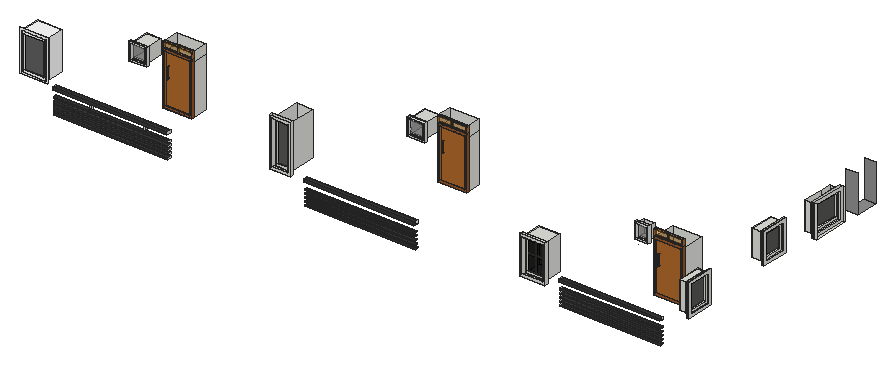
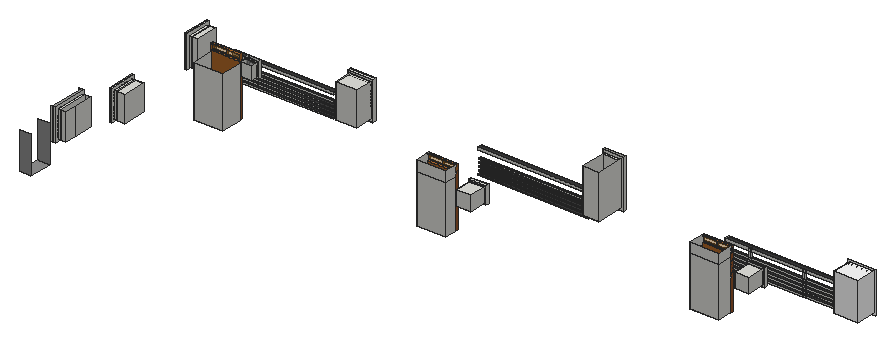
# SketchUp Ruby script. Lengths in inches.
U = 1.inch
M = Sketchup.active_model
def pt(a) = Geom::Point3d.new(a.map { |v| v * U })
def face(e, loops, mat)
  f = e.add_face(loops[0].map { |a| pt(a) })
  loops[1..].each { |l| e.add_face(l.map { |a| pt(a) }).erase! }
  f.material = f.back_material = mat if mat
  f
end
# faces: each face lists its corners as indices into pts; further lists are holes
def faces(e, pts, list, mat = nil) = list.each { |f| face(e, (f[0].is_a?(Array) ? f : [f]).map { |l| l.map { |i| pts[i] } }, mat) }
# xy, xz, yz: faces in a plane at the given z, y or x. An outline is a flat list of corners, or four numbers for a rectangle; further outlines are holes
def ring(l) = l.size == 4 ? [[l[0], l[1]], [l[2], l[1]], [l[2], l[3]], [l[0], l[3]]] : l.each_slice(2).to_a
def flat(e, list, mat, &to3) = list.each { |f| face(e, (f[0].is_a?(Array) ? f : [f]).map { |l| ring(l).map { |u, v| to3.(u, v) } }, mat) }
def xy(e, z, list, mat = nil) = flat(e, list, mat) { |x, y| [x, y, z] }
def xz(e, y, list, mat = nil) = flat(e, list, mat) { |x, z| [x, y, z] }
def yz(e, x, list, mat = nil) = flat(e, list, mat) { |y, z| [x, y, z] }
def lines(e, pts, list) = list.each { |a, b| e.add_line(pt(pts[a]), pt(pts[b])) }
# prism: a flat outline (further loops are holes) pulled along v
def prism(e, loops, v, mat = nil)
  f = face(e, loops, mat); d = Geom::Vector3d.new(v.map { |x| x * U })
  f.pushpull(f.normal.samedirection?(d) ? d.length : -d.length)
end
def box(e, o, s, mat = nil) = prism(e, [[o, [o[0] + s[0], o[1], o[2]], [o[0] + s[0], o[1] + s[1], o[2]], [o[0], o[1] + s[1], o[2]]]], [0, 0, s[2]], mat)
def at(x, y, z, deg = 0) = Geom::Transformation.translation(pt([x, y, z])) * Geom::Transformation.rotation(ORIGIN, Z_AXIS, deg.degrees)
def axes(o, x, y, z) = Geom::Transformation.new([*x, 0, *y, 0, *z, 0, *pt(o).to_a, 1])
def part(name) = M.definitions.add(name)
# library, detail: a bought-in or finely detailed component or shape, given as its bounding box
def library(name, o, s) = part(name).tap { |d| box(d.entities, o, s) }
def detail(e, o, s) = box(e.add_group.entities, o, s)
def put(e, d, t, mat = nil) = e.add_instance(d, t).tap { |i| i.material = mat if mat }
def group(e, t, mat = nil) = e.add_group.tap { |g| g.transformation = t; g.material = mat if mat }.entities
root = M.entities
M.materials.add("Generic").color = [145, 145, 145]
M.materials.add("[Color M00]").color = [255, 255, 255]
M.materials.add("[Color M07]").color = [58, 58, 58]
M.materials.add("[Color M08]").color = [45, 45, 45]
M.materials.add("[Translucent Glass Dark Green]").color = [168, 100, 12]
M.materials["[Translucent Glass Dark Green]"].alpha = 0.5
M.materials.add("[Translucent Glass Gray]").color = [0, 0, 0]
M.materials["[Translucent Glass Gray]"].alpha = 0.62
M.materials.add("[Translucent Glass Gray]1").color = [128, 128, 128]
M.materials["[Translucent Glass Gray]1"].alpha = 0.5
M.materials.add("[Wood Bamboo]").color = [177, 105, 43]
M.materials.add("[Wood Cherry Original]").color = [152, 86, 42]
c1 = part("Group\#10")
xy(c1.entities,0,[[0,1.08,55.8125,6.01]],"[Wood Cherry Original]")
xy(c1.entities,3.96,[[3.96,1.08,51.86,3.01]],"[Wood Bamboo]")
xy(c1.entities,51.66,[[8.63,0,9.88,3.01]],"[Color M08]")
xy(c1.entities,52.54,[[8.63,0.6875,9.88,3.01]],"[Color M08]")
xy(c1.entities,71.82,[[8.63,0.6875,9.88,3.01]],"[Color M08]")
xy(c1.entities,72.69,[[8.63,0,9.88,3.01]],"[Color M08]")
xy(c1.entities,97.36,[[3.96,1.08,51.86,3.01]],"[Wood Bamboo]")
xy(c1.entities,101.3125,[[0,1.08,55.8125,6.01]],"[Wood Bamboo]")
xy(c1.entities,102.55,[[1.23,1.08,27.29,3.01],[27.29,1.08,28.52,1.95],[28.52,1.08,54.58,3.01]],"[Wood Bamboo]")
xy(c1.entities,112.31,[[1.23,1.08,1.23,3.01,27.29,3.01,27.29,1.95,28.52,1.95,28.52,3.01,54.58,3.01,54.58,1.08]],"[Wood Bamboo]")
xy(c1.entities,113.54,[[0,1.08,55.8125,6.01]],"[Wood Bamboo]")
xz(c1.entities,0,[[8.63,51.66,9.88,72.69]],"[Color M08]")
xz(c1.entities,0.6875,[[8.63,52.54,9.88,71.82]])
xz(c1.entities,1.08,[[0,101.3125,55.8125,102.55],[0,102.55,1.23,102.55,1.23,112.31,54.58,112.31,54.58,102.55,55.8125,102.55,55.8125,113.54,0,113.54]],"[Wood Bamboo]")
xz(c1.entities,1.08,[[[0,0,55.8125,101.3125],[3.96,3.96,51.86,97.36]]],"[Wood Cherry Original]")
xz(c1.entities,1.95,[[27.29,102.55,28.52,112.31]],"[Wood Bamboo]")
xz(c1.entities,3.01,[[8.63,71.82,9.88,72.69]])
xz(c1.entities,3.01,[[1.23,102.55,27.29,112.31],[28.52,102.55,54.58,112.31]],"[Translucent Glass Dark Green]")
xz(c1.entities,3.01,[[[3.96,3.96,51.86,97.36],[8.63,71.82,9.88,72.69],[8.63,51.66,9.88,52.54]]],"[Wood Bamboo]")
xz(c1.entities,6.01,[[0,0,55.8125,101.3125],[0,112.31,55.8125,113.54]],"[Wood Bamboo]")
yz(c1.entities,0,[[1.08,101.3125,6.01,113.54]],"[Wood Bamboo]")
yz(c1.entities,0,[[1.08,0,6.01,101.3125]],"[Wood Cherry Original]")
yz(c1.entities,1.23,[[1.08,102.55,3.01,112.31]],"[Wood Bamboo]")
yz(c1.entities,3.96,[[1.08,3.96,3.01,97.36]],"[Wood Bamboo]")
yz(c1.entities,8.63,[[0,51.66,0,72.69,3.01,72.69,3.01,71.82,0.6875,71.82,0.6875,52.54,3.01,52.54,3.01,51.66]],"[Color M08]")
yz(c1.entities,9.88,[[0,51.66,3.01,51.66,3.01,52.54,0.6875,52.54,0.6875,71.82,3.01,71.82,3.01,72.69,0,72.69]],"[Color M08]")
yz(c1.entities,27.29,[[1.95,102.55,3.01,112.31]],"[Wood Bamboo]")
yz(c1.entities,28.52,[[1.95,102.55,3.01,112.31]],"[Wood Bamboo]")
yz(c1.entities,51.86,[[1.08,3.96,3.01,97.36]],"[Wood Bamboo]")
yz(c1.entities,54.58,[[1.08,102.55,3.01,112.31]],"[Wood Bamboo]")
yz(c1.entities,55.8125,[[1.08,101.3125,6.01,113.54]],"[Wood Bamboo]")
yz(c1.entities,55.8125,[[1.08,0,6.01,101.3125]],"[Wood Cherry Original]")
p = [[1.23,3.01,112.31],[1.23,6.01,112.31],[9.24,3.01,71.99],[9.24,0.51,71.99],[9.24,0.51,52.37],[9.24,3.01,52.37]]
lines(c1.entities,p,[[0,1],[2,3],[3,4],[4,5]])
c2 = part("Group\#1")
xy(c2.entities,0,[[0,0,39.9375,6]])
xy(c2.entities,3.79,[[3.79,0,36.15,3]])
xy(c2.entities,60.83,[[3.79,0,36.15,3]])
xy(c2.entities,64.62,[[0,0,39.9375,6]])
xz(c2.entities,0,[[[0,0,39.9375,64.62],[3.79,3.79,36.15,60.83]]])
xz(c2.entities,3,[[18.07,3.79,20.49,3.79,20.49,32.1,36.15,32.1,36.15,34.21,20.49,34.21,20.49,60.83,18.07,60.83,18.07,34.21,3.79,34.21,3.79,32.1,18.07,32.1]],"[Color M08]")
xz(c2.entities,3,[[3.79,3.79,18.07,32.1],[20.49,3.79,36.15,32.1],[3.79,34.21,18.07,60.83],[20.49,34.21,36.15,60.83]],"[Translucent Glass Gray]")
xz(c2.entities,6,[[0,0,39.9375,64.62]],"[Translucent Glass Gray]")
yz(c2.entities,0,[[0,0,6,64.62]])
yz(c2.entities,3.79,[[0,3.79,3,60.83]])
yz(c2.entities,36.15,[[0,3.79,3,60.83]])
yz(c2.entities,39.9375,[[0,0,6,64.62]])
c3 = part("Group\#5")
xy(c3.entities,0,[[0,0,46.6875,6]],"[Color M00]")
xy(c3.entities,4.48,[[4.48,0,42.2,3]],"[Color M00]")
xy(c3.entities,67.45,[[4.48,0,42.2,3]],"[Color M00]")
xy(c3.entities,71.9375,[[0,0,46.6875,6]],"[Color M00]")
xz(c3.entities,0,[[[0,0,46.6875,71.9375],[4.48,4.48,42.2,67.45]]],"[Color M00]")
xz(c3.entities,3,[[4.48,4.48,42.2,67.45]],"[Translucent Glass Gray]")
xz(c3.entities,6,[[0,0,46.6875,71.9375]],"[Color M00]")
yz(c3.entities,0,[[0,0,6,71.9375]],"[Color M00]")
yz(c3.entities,4.48,[[0,4.48,3,67.45]],"[Color M00]")
yz(c3.entities,42.2,[[0,4.48,3,67.45]],"[Color M00]")
yz(c3.entities,46.6875,[[0,0,6,71.9375]],"[Color M00]")
c4 = part("Group\#3")
xy(c4.entities,0,[[0,0,31.25,5.5]])
xy(c4.entities,4.35,[[4.35,0,26.9,2.5]])
xy(c4.entities,79.53,[[4.35,0,26.9,2.5]])
xy(c4.entities,83.875,[[0,0,31.25,5.5]])
xz(c4.entities,0,[[[0,0,31.25,83.875],[4.35,4.35,26.9,79.53]]])
xz(c4.entities,2.5,[[4.35,4.35,26.9,79.53]],"[Translucent Glass Gray]")
xz(c4.entities,5.5,[[0,0,31.25,83.875]])
yz(c4.entities,0,[[0,0,5.5,83.875]])
yz(c4.entities,4.35,[[0,4.35,2.5,79.53]])
yz(c4.entities,26.9,[[0,4.35,2.5,79.53]])
yz(c4.entities,31.25,[[0,0,5.5,83.875]])
c5 = part("Group\#7")
xy(c5.entities,0,[[0,0,6,43.1875]])
xy(c5.entities,3.45,[[3,3.45,6,39.74]])
xy(c5.entities,49.61,[[3,3.45,6,39.74]])
xy(c5.entities,53.0625,[[0,0,6,43.1875]])
xz(c5.entities,0,[[0,0,6,53.0625]])
xz(c5.entities,3.45,[[3,3.45,6,49.61]])
xz(c5.entities,39.74,[[3,3.45,6,49.61]])
xz(c5.entities,43.1875,[[0,0,6,53.0625]])
yz(c5.entities,0,[[0,0,43.1875,53.0625]])
yz(c5.entities,3,[[3.45,3.45,39.74,49.61]],"[Translucent Glass Gray]")
yz(c5.entities,6,[[[0,0,43.1875,53.0625],[3.45,3.45,39.74,49.61]]])
c6 = part("Group\#6")
xy(c6.entities,0,[[0,0,6,44.5]])
xy(c6.entities,4.57,[[3,4.57,6,39.93]])
xy(c6.entities,45.43,[[3,4.57,6,39.93]])
xy(c6.entities,50,[[0,0,6,44.5]])
xz(c6.entities,0,[[0,0,6,50]])
xz(c6.entities,4.57,[[3,4.57,6,45.43]])
xz(c6.entities,39.93,[[3,4.57,6,45.43]])
xz(c6.entities,44.5,[[0,0,6,50]])
yz(c6.entities,0,[[0,0,44.5,50]])
yz(c6.entities,3,[[4.57,4.57,39.93,45.43]],"[Translucent Glass Gray]")
yz(c6.entities,6,[[[0,0,44.5,50],[4.57,4.57,39.93,45.43]]])
c7 = part("Group\#8")
xy(c7.entities,0,[[0,0,6,59.4375]])
xy(c7.entities,4.64,[[3,4.64,6,54.8]])
xy(c7.entities,46.99,[[3,4.64,6,54.8]])
xy(c7.entities,51.625,[[0,0,6,59.4375]])
xz(c7.entities,0,[[0,0,6,51.625]])
xz(c7.entities,4.64,[[3,4.64,6,46.99]])
xz(c7.entities,54.8,[[3,4.64,6,46.99]])
xz(c7.entities,59.4375,[[0,0,6,51.625]])
yz(c7.entities,0,[[0,0,59.4375,51.625]])
yz(c7.entities,3,[[4.64,4.64,54.8,46.99]],"[Translucent Glass Gray]")
yz(c7.entities,6,[[[0,0,59.4375,51.625],[4.64,4.64,54.8,46.99]]])
c8 = part("Group\#11")
xy(c8.entities,0,[[0,0,27.8125,3]])
xy(c8.entities,27.8125,[[0,0,27.8125,3]])
xz(c8.entities,0,[[0,0,27.8125,27.8125]],"[Translucent Glass Gray]1")
xz(c8.entities,3,[[0,0,27.8125,27.8125]],"[Translucent Glass Gray]1")
yz(c8.entities,0,[[0,0,3,27.8125]])
yz(c8.entities,27.8125,[[0,0,3,27.8125]])
c9 = part("Group\#12")
xy(c9.entities,0,[[0,0,20.25,3]])
xy(c9.entities,24.8125,[[0,0,20.25,3]])
xz(c9.entities,0,[[0,0,20.25,24.8125]],"[Translucent Glass Gray]1")
xz(c9.entities,3,[[0,0,20.25,24.8125]],"[Translucent Glass Gray]1")
yz(c9.entities,0,[[0,0,3,24.8125]])
yz(c9.entities,20.25,[[0,0,3,24.8125]])
xy(root,394.36,[[272.78,74.79,492.5625,80.4375]],"[Color M07]")
xy(root,394.51,[[1230.96,91.08,1423.39,96.64]],"[Color M07]")
xy(root,395.27,[[741.96,90.52,954.11,95.33]],"[Color M07]")
xy(root,397.15,[[741.96,90.52,954.11,95.33]],"[Color M07]")
xy(root,397.26,[[1230.96,91.08,1423.39,96.64]],"[Color M07]")
xy(root,397.74,[[272.78,74.79,492.5625,80.4375]],"[Color M07]")
xy(root,399.1875,[[392.26,187.125,448.07,220.9375]])
xy(root,401.51,[[1230.96,91.08,1423.39,96.64]],"[Color M07]")
xy(root,401.61,[[272.78,74.79,492.5625,80.4375]],"[Color M07]")
xy(root,401.9,[[741.96,90.27,954.11,95.08]],"[Color M07]")
xy(root,403.35,[[1327.46,199.25,1383.27,240]])
xy(root,403.77,[[741.96,90.27,954.11,95.08]],"[Color M07]")
xy(root,404.26,[[1230.96,91.08,1423.39,96.64]],"[Color M07]")
xy(root,404.99,[[272.78,74.79,492.5625,80.4375]],"[Color M07]")
xy(root,405.73,[[862.05,258.8125,917.86,288.3125]])
xy(root,408.18,[[272.78,74.79,492.5625,80.4375]],"[Color M07]")
xy(root,408.7,[[1230.96,91.08,1423.39,96.64]],"[Color M07]")
xy(root,408.77,[[741.96,90.33,954.11,95.14]],"[Color M07]")
xy(root,410.65,[[741.96,90.33,954.11,95.14]],"[Color M07]")
xy(root,411.45,[[1230.96,91.08,1423.39,96.64]],"[Color M07]")
xy(root,411.55,[[272.78,74.79,492.5625,80.4375]],"[Color M07]")
xy(root,415.24,[[272.78,74.79,492.5625,80.4375]],"[Color M07]")
xy(root,415.32,[[1230.96,91.08,1423.39,96.64]],"[Color M07]")
xy(root,416.28,[[741.96,90.27,954.11,95.08]],"[Color M07]")
xy(root,418.07,[[1151.9,93.8125,1200.57,99.8125]])
xy(root,418.07,[[1230.96,91.08,1423.39,96.64]],"[Color M07]")
xy(root,418.16,[[741.96,90.27,954.11,95.08]],"[Color M07]")
xy(root,418.62,[[272.78,74.79,492.5625,80.4375]],"[Color M07]")
xy(root,422.31,[[272.78,74.79,492.5625,80.4375]],"[Color M07]")
xy(root,422.44,[[1156.27,93.8125,1196.2,99.8125],[1156.27,99.8125,1196.2,134.3125]])
xy(root,422.82,[[1230.96,91.08,1423.39,96.64]],"[Color M07]")
xy(root,422.85,[[741.96,90.39,954.11,95.2]],"[Color M07]")
xy(root,424.72,[[741.96,90.39,954.11,95.2]],"[Color M07]")
xy(root,425.57,[[1230.96,91.08,1423.39,96.64]],"[Color M07]")
xy(root,425.68,[[272.78,74.79,492.5625,80.4375]],"[Color M07]")
xy(root,428.35,[[192.03,99.8125,238.71,138.75]],"[Color M00]")
xy(root,433.8,[[672.35,93.8125,712.33,99.8125]])
xy(root,436.87,[[1429.21,528.77,1451.02,572.96]],"Generic")
xy(root,437.05,[[1448.83,123.62,1452.83,175.61]])
xy(root,437.21,[[1435.83,318.51,1439.83,371.82]])
xy(root,437.21,[[1230.96,88.89,1423.39,96.64]],"[Color M07]")
xy(root,437.31,[[272.78,72.41,492.5625,80.4375]],"[Color M07]")
xy(root,437.85,[[741.96,87.39,954.11,95.33]],"[Color M07]")
xy(root,438.17,[[676.72,93.8125,707.97,99.8125],[676.72,99.8125,707.97,152.375]])
xy(root,438.37,[[442.43,76.97,444,80.4375]])
xy(root,441.06,[[445.18,76.97,446.75,80.4375]])
xy(root,441.31,[[339.06,76.97,340.62,80.4375],[341.81,76.97,343.37,80.4375]])
xy(root,441.45,[[1430.27,128.02,1448.83,171.21],[1448.83,128.02,1452.83,171.21]])
xy(root,441.61,[[1414.21,322.92,1435.83,367.42],[1435.83,322.92,1439.83,367.42]])
xy(root,442.14,[[1230.96,88.89,1423.39,96.64]],"[Color M07]")
xy(root,442.24,[[272.78,72.41,492.5625,80.4375]],"[Color M07]")
xy(root,443.28,[[741.96,87.39,954.11,95.33]],"[Color M07]")
xy(root,447.34,[[1452.58,417.16,1457.58,485.41],[1457.58,417.16,1462.21,485.41]])
xy(root,451.74,[[1435.83,421.57,1452.58,481],[1452.58,421.57,1457.58,481]])
xy(root,461.13,[[331.98,182.0625,365.3125,187.125]])
xy(root,463.88,[[334.74,182.0625,362.55,187.125],[334.74,187.125,362.55,221.125]])
xy(root,467.09,[[808.05,253.75,841.375,258.8125]])
xy(root,469.85,[[810.81,253.75,838.62,258.8125],[810.81,258.8125,838.62,292.8125]])
xy(root,486.72,[[1292.01,194.1875,1317.77,199.25]])
xy(root,487.0625,[[1156.27,93.8125,1196.2,99.8125],[1156.27,99.8125,1196.2,134.3125]])
xy(root,489.48,[[1294.76,194.1875,1315.01,199.25],[1294.76,199.25,1315.01,212.4375]])
xy(root,491.43,[[1151.9,93.8125,1200.57,99.8125]])
xy(root,491.61,[[1414.21,322.92,1435.83,367.42],[1435.83,322.92,1439.83,367.42]])
xy(root,491.7,[[334.74,182.0625,362.55,187.125],[334.74,187.125,362.55,221.125]])
xy(root,494.45,[[331.98,182.0625,365.3125,187.125]])
xy(root,494.51,[[1430.27,128.02,1448.83,171.21],[1448.83,128.02,1452.83,171.21]])
xy(root,496.01,[[1435.83,318.51,1439.83,371.82]])
xy(root,497.66,[[810.81,253.75,838.62,258.8125],[810.81,258.8125,838.62,292.8125]])
xy(root,498.92,[[1448.83,123.62,1452.83,175.61]])
xy(root,500.29,[[192.03,99.8125,238.71,138.75]],"[Color M00]")
xy(root,500.42,[[808.05,253.75,841.375,258.8125]])
xz(root,72.41,[[272.78,437.31,492.5625,442.24]],"[Color M07]")
xz(root,74.79,[[272.78,394.36,492.5625,397.74],[272.78,401.61,492.5625,404.99],[272.78,408.18,492.5625,411.55],[272.78,415.24,492.5625,418.62],[272.78,422.31,492.5625,425.68]],"[Color M07]")
xz(root,80.4375,[[272.78,394.36,339.06,397.74],[339.06,394.36,340.62,397.74],[340.62,394.36,341.81,397.74],[341.81,394.36,343.37,397.74],[343.37,394.36,442.43,397.74],
  [442.43,394.36,444,397.74],[444,394.36,445.18,397.74],[445.18,394.36,446.75,397.74],[446.75,394.36,492.5625,397.74],[339.06,397.74,340.62,401.61],
  [341.81,397.74,343.37,401.61],[442.43,397.74,444,401.61],[445.18,397.74,446.75,401.61],[272.78,401.61,339.06,404.99],[339.06,401.61,340.62,404.99],
  [340.62,401.61,341.81,404.99],[341.81,401.61,343.37,404.99],[343.37,401.61,442.43,404.99],[442.43,401.61,444,404.99],[444,401.61,445.18,404.99],
  [445.18,401.61,446.75,404.99],[446.75,401.61,492.5625,404.99],[339.06,404.99,340.62,408.18],[341.81,404.99,343.37,408.18],[442.43,404.99,444,408.18],
  [445.18,404.99,446.75,408.18],[272.78,408.18,339.06,411.55],[339.06,408.18,340.62,411.55],[340.62,408.18,341.81,411.55],[341.81,408.18,343.37,411.55],
  [343.37,408.18,442.43,411.55],[442.43,408.18,444,411.55],[444,408.18,445.18,411.55],[445.18,408.18,446.75,411.55],[446.75,408.18,492.5625,411.55],
  [339.06,411.55,340.62,415.24],[341.81,411.55,343.37,415.24],[442.43,411.55,444,415.24],[445.18,411.55,446.75,415.24],[272.78,415.24,339.06,418.62],
  [339.06,415.24,340.62,418.62],[340.62,415.24,341.81,418.62],[341.81,415.24,343.37,418.62],[343.37,415.24,442.43,418.62],[442.43,415.24,444,418.62],
  [444,415.24,445.18,418.62],[445.18,415.24,446.75,418.62],[446.75,415.24,492.5625,418.62],[339.06,418.62,340.62,422.31],[341.81,418.62,343.37,422.31],
  [442.43,418.62,444,422.31],[445.18,418.62,446.75,422.31],[272.78,422.31,339.06,425.68],[339.06,422.31,340.62,425.68],[340.62,422.31,341.81,425.68],
  [341.81,422.31,343.37,425.68],[343.37,422.31,442.43,425.68],[442.43,422.31,444,425.68],[444,422.31,445.18,425.68],[445.18,422.31,446.75,425.68],
  [446.75,422.31,492.5625,425.68],[339.06,425.68,340.62,437.31],[341.81,425.68,343.37,437.31],[442.43,425.68,444,437.31],[445.18,425.68,446.75,437.31],
  [272.78,437.31,339.06,442.24],[339.06,437.31,340.62,441.31],[340.62,437.31,341.81,442.24],[341.81,437.31,343.37,441.31],[343.37,437.31,442.43,442.24],
  [442.43,437.31,444,438.37],[444,437.31,444,442.24,492.5625,442.24,492.5625,437.31,446.75,437.31,446.75,441.06,445.18,441.06,445.18,437.31],[445.18,437.31,446.75,441.06],[442.43,438.37,444,442.24],[339.06,441.31,340.62,442.24],
  [341.81,441.31,343.37,442.24]])
xz(root,87.39,[[741.96,437.85,954.11,443.28]],"[Color M07]")
xz(root,88.89,[[1230.96,437.21,1423.39,442.14]],"[Color M07]")
xz(root,90.27,[[741.96,401.9,954.11,403.77],[741.96,416.28,954.11,418.16]],"[Color M07]")
xz(root,90.33,[[741.96,408.77,954.11,410.65]],"[Color M07]")
xz(root,90.39,[[741.96,422.85,954.11,424.72]],"[Color M07]")
xz(root,90.52,[[741.96,395.27,954.11,397.15]],"[Color M07]")
xz(root,91.08,[[1230.96,394.51,1423.39,397.26],[1230.96,401.51,1423.39,404.26],[1230.96,408.7,1423.39,411.45],[1230.96,415.32,1423.39,418.07],[1230.96,422.82,1423.39,425.57]],"[Color M07]")
xz(root,93.8125,[[[1151.9,418.07,1200.57,491.43],[1156.27,422.44,1196.2,487.0625]],[[672.35,433.8,712.33,526.41],[676.72,438.17,707.97,522.04]]])
xz(root,95.08,[[741.96,401.9,954.11,403.77],[741.96,416.28,954.11,418.16]])
xz(root,95.14,[[741.96,408.77,954.11,410.65]])
xz(root,95.2,[[741.96,422.85,954.11,424.72]])
xz(root,95.33,[[741.96,395.27,954.11,397.15],[741.96,437.85,954.11,443.28]])
xz(root,96.64,[[1230.96,394.51,1423.39,397.26],[1230.96,401.51,1423.39,404.26],[1230.96,408.7,1423.39,411.45],[1230.96,415.32,1423.39,418.07],[1230.96,422.82,1423.39,425.57],
  [1230.96,437.21,1423.39,442.14]])
xz(root,99.8125,[[[1151.9,418.07,1200.57,491.43],[1156.27,422.44,1196.2,487.0625]],[[672.35,433.8,712.33,526.41],[676.72,438.17,707.97,522.04]]])
xz(root,99.8125,[[[188.42,424.75,242.3125,503.89],[192.03,428.35,238.71,500.29]]],"[Color M00]")
xz(root,123.62,[[1448.83,437.05,1452.83,498.92]])
xz(root,128.02,[[1430.27,441.45,1448.83,494.51],[1448.83,441.45,1452.83,494.51]])
xz(root,134.3125,[[1156.27,422.44,1196.2,487.0625]])
xz(root,138.75,[[192.03,428.35,238.71,500.29]],"[Color M00]")
xz(root,152.375,[[676.72,438.17,707.97,522.04]])
xz(root,171.21,[[1430.27,441.45,1448.83,494.51],[1448.83,441.45,1452.83,494.51]])
xz(root,175.61,[[1448.83,437.05,1452.83,498.92]])
xz(root,182.0625,[[[331.98,461.13,365.3125,494.45],[334.74,463.88,362.55,491.7]]])
xz(root,187.125,[[[331.98,461.13,365.3125,494.45],[334.74,463.88,362.55,491.7]]])
xz(root,194.1875,[[[1292.01,486.72,1317.77,517.05],[1294.76,489.48,1315.01,514.29]]])
xz(root,199.25,[[[1292.01,486.72,1317.77,517.05],[1294.76,489.48,1315.01,514.29]]])
xz(root,212.4375,[[1294.76,489.48,1315.01,514.29]])
xz(root,220.9375,[[392.26,399.1875,448.07,493.72],[392.26,493.72,448.07,512.73]])
xz(root,221.125,[[334.74,463.88,362.55,491.7]])
xz(root,240,[[1327.46,403.35,1383.27,501.62]])
xz(root,253.75,[[[808.05,467.09,841.375,500.42],[810.81,469.85,838.62,497.66]]])
xz(root,258.8125,[[[808.05,467.09,841.375,500.42],[810.81,469.85,838.62,497.66]]])
xz(root,288.3125,[[862.05,405.73,917.86,498.87],[862.05,498.87,917.86,519.27]])
xz(root,292.8125,[[810.81,469.85,838.62,497.66]])
xz(root,318.51,[[1435.83,437.21,1439.83,496.01]])
xz(root,322.92,[[1414.21,441.61,1435.83,491.61],[1435.83,441.61,1439.83,491.61]])
xz(root,367.42,[[1414.21,441.61,1435.83,491.61],[1435.83,441.61,1439.83,491.61]])
xz(root,371.82,[[1435.83,437.21,1439.83,496.01]])
xz(root,417.16,[[1452.58,447.34,1457.58,507.77],[1457.58,447.34,1462.21,507.77]])
xz(root,421.57,[[1435.83,451.74,1452.58,503.36],[1452.58,451.74,1457.58,503.36]])
xz(root,481,[[1435.83,451.74,1452.58,503.36],[1452.58,451.74,1457.58,503.36]])
xz(root,485.41,[[1452.58,447.34,1457.58,507.77],[1457.58,447.34,1462.21,507.77]])
xz(root,528.77,[[1429.21,436.87,1451.02,508.37]],"Generic")
xz(root,572.96,[[1429.21,436.87,1451.02,508.37]],"Generic")
yz(root,192.03,[[99.8125,428.35,138.75,500.29]],"[Color M00]")
yz(root,238.71,[[99.8125,428.35,138.75,500.29]],"[Color M00]")
yz(root,272.78,[[74.79,394.36,80.4375,397.74],[74.79,401.61,80.4375,404.99],[74.79,408.18,80.4375,411.55],[74.79,415.24,80.4375,418.62],[74.79,422.31,80.4375,425.68],
  [72.41,437.31,80.4375,442.24]])
yz(root,331.98,[[182.0625,461.13,187.125,494.45]])
yz(root,334.74,[[182.0625,463.88,187.125,491.7],[187.125,463.88,221.125,491.7]])
yz(root,362.55,[[182.0625,463.88,187.125,491.7],[187.125,463.88,221.125,491.7]])
yz(root,365.3125,[[182.0625,461.13,187.125,494.45]])
yz(root,392.26,[[187.125,399.1875,220.9375,493.72],[187.125,493.72,220.9375,512.73]])
yz(root,448.07,[[187.125,399.1875,220.9375,493.72],[187.125,493.72,220.9375,512.73]])
yz(root,492.5625,[[74.79,394.36,80.4375,397.74],[74.79,401.61,80.4375,404.99],[74.79,408.18,80.4375,411.55],[74.79,415.24,80.4375,418.62],[74.79,422.31,80.4375,425.68],
  [72.41,437.31,80.4375,442.24]])
yz(root,672.35,[[93.8125,433.8,99.8125,526.41]])
yz(root,676.72,[[93.8125,438.17,99.8125,522.04],[99.8125,438.17,152.375,522.04]])
yz(root,707.97,[[93.8125,438.17,99.8125,522.04],[99.8125,438.17,152.375,522.04]])
yz(root,712.33,[[93.8125,433.8,99.8125,526.41]])
yz(root,741.96,[[90.52,395.27,95.33,397.15],[90.27,401.9,95.08,403.77],[90.33,408.77,95.14,410.65],[90.27,416.28,95.08,418.16],[90.39,422.85,95.2,424.72],
  [87.39,437.85,95.33,443.28]])
yz(root,808.05,[[253.75,467.09,258.8125,500.42]])
yz(root,810.81,[[253.75,469.85,258.8125,497.66],[258.8125,469.85,292.8125,497.66]])
yz(root,838.62,[[253.75,469.85,258.8125,497.66],[258.8125,469.85,292.8125,497.66]])
yz(root,841.375,[[253.75,467.09,258.8125,500.42]])
yz(root,862.05,[[258.8125,405.73,288.3125,498.87],[258.8125,498.87,288.3125,519.27]])
yz(root,917.86,[[258.8125,405.73,288.3125,498.87],[258.8125,498.87,288.3125,519.27]])
yz(root,1151.9,[[93.8125,418.07,99.8125,491.43]])
yz(root,1156.27,[[93.8125,422.44,99.8125,487.0625],[99.8125,422.44,134.3125,487.0625]])
yz(root,1196.2,[[93.8125,422.44,99.8125,487.0625],[99.8125,422.44,134.3125,487.0625]])
yz(root,1200.57,[[93.8125,418.07,99.8125,491.43]])
yz(root,1230.96,[[91.08,394.51,96.64,397.26],[91.08,401.51,96.64,404.26],[91.08,408.7,96.64,411.45],[91.08,415.32,96.64,418.07],[91.08,422.82,96.64,425.57],
  [88.89,437.21,96.64,442.14]])
yz(root,1292.01,[[194.1875,486.72,199.25,517.05]])
yz(root,1294.76,[[194.1875,489.48,199.25,514.29],[199.25,489.48,212.4375,514.29]])
yz(root,1315.01,[[194.1875,489.48,199.25,514.29],[199.25,489.48,212.4375,514.29]])
yz(root,1317.77,[[194.1875,486.72,199.25,517.05]])
yz(root,1327.46,[[199.25,403.35,240,501.62]])
yz(root,1383.27,[[199.25,403.35,240,501.62]])
yz(root,1414.21,[[322.92,441.61,367.42,491.61]])
yz(root,1430.27,[[128.02,441.45,171.21,494.51]])
yz(root,1435.83,[[[318.51,437.21,371.82,496.01],[322.92,441.61,367.42,491.61]],[421.57,451.74,459.8125,503.36],[459.8125,451.74,481,503.36]])
yz(root,1439.83,[[[318.51,437.21,371.82,496.01],[322.92,441.61,367.42,491.61]]])
yz(root,1448.83,[[[123.62,437.05,175.61,498.92],[128.02,441.45,171.21,494.51]]])
yz(root,1452.58,[[[417.16,447.34,485.41,507.77],[421.57,451.74,481,503.36]]])
yz(root,1452.83,[[[123.62,437.05,175.61,498.92],[128.02,441.45,171.21,494.51]]])
yz(root,1457.58,[[[417.16,447.34,485.41,507.77],[421.57,451.74,481,503.36]]])
p = [[272.78,77.5,396],[482.8125,77.5,396],[272.78,77.5,403],[482.8125,77.5,403],[272.78,77.5,410],[482.8125,77.5,410],
  [272.78,77.5,417],[482.8125,77.5,417],[272.78,77.5,424],[482.8125,77.5,424],[272.78,77.5,439],[482.8125,77.5,439],
  [444,76.97,438.37],[444,76.97,442.24],[741.96,92.91,396],[954.11,92.91,396],[741.96,92.91,403],[954.11,92.91,403],
  [741.96,92.91,410],[954.11,92.91,410],[741.96,92.91,417],[954.11,92.91,417],[741.96,92.91,424],[954.11,92.91,424],
  [741.96,92.91,439],[954.11,92.91,439],[1230.96,93.91,396],[1423.39,93.91,396],[1230.96,93.91,403],[1423.39,93.91,403],
  [1230.96,93.91,410],[1423.39,93.91,410],[1230.96,93.91,417],[1423.39,93.91,417],[1230.96,93.91,424],[1423.39,93.91,424],
  [1230.96,93.91,439],[1423.39,93.91,439],[1295.17,199.25,476.08],[1295.23,199.25,476.08]]
lines(root,p,[[0,1],[2,3],[4,5],[6,7],[8,9],[10,11],[12,13],[14,15],[16,17],[18,19],[20,21],[22,23],
  [24,25],[26,27],[28,29],[30,31],[32,33],[34,35],[36,37],[38,39]])
put(root,c1,at(392.26,187.125,399.1875))
put(root,c1,at(1327.46,193.24,403.35))
put(root,c1,at(862.05,257.74,405.73))
put(root,c2,at(1156.27,99.8125,422.44))
put(root,c3,at(192.03,99.8125,428.35))
put(root,c4,at(676.72,99.8125,438.17))
put(root,c5,at(1442.83,128.02,441.45))
put(root,c6,at(1429.83,322.92,441.61))
put(root,c7,at(1446.58,421.57,451.74))
put(root,c8,at(334.74,187.125,463.88))
put(root,c8,at(810.81,258.8125,469.85))
put(root,c9,at(1294.76,199.25,489.48))
